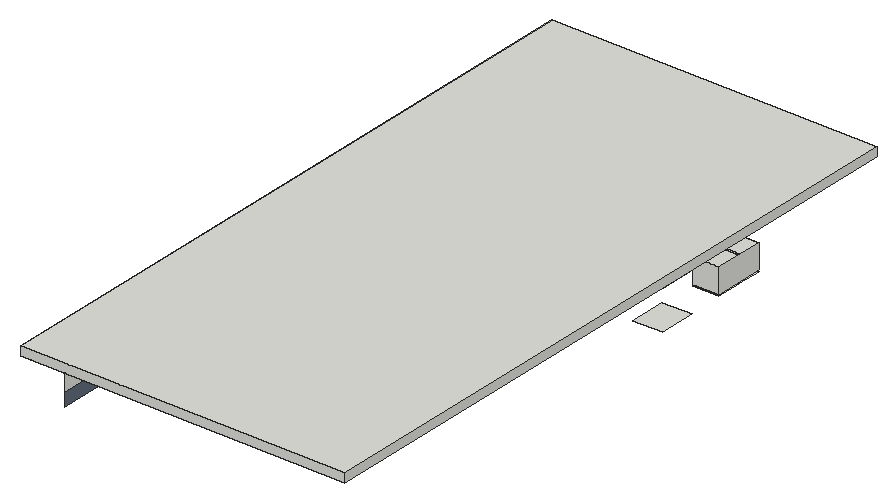
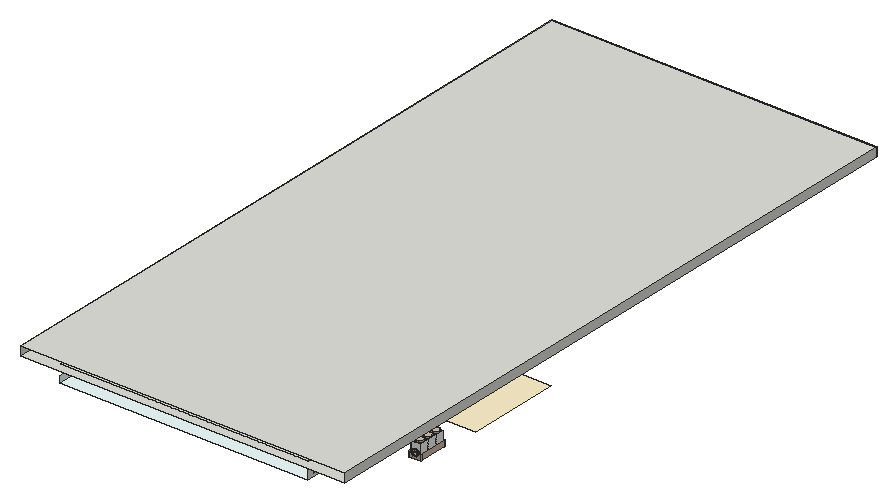
# SketchUp Ruby script. Lengths in inches.
U = 1.inch
M = Sketchup.active_model
def pt(a) = Geom::Point3d.new(a.map { |v| v * U })
def face(e, loops, mat)
  f = e.add_face(loops[0].map { |a| pt(a) })
  loops[1..].each { |l| e.add_face(l.map { |a| pt(a) }).erase! }
  f.material = f.back_material = mat if mat
  f
end
# faces: each face lists its corners as indices into pts; further lists are holes
def faces(e, pts, list, mat = nil) = list.each { |f| face(e, (f[0].is_a?(Array) ? f : [f]).map { |l| l.map { |i| pts[i] } }, mat) }
# xy, xz, yz: faces in a plane at the given z, y or x. An outline is a flat list of corners, or four numbers for a rectangle; further outlines are holes
def ring(l) = l.size == 4 ? [[l[0], l[1]], [l[2], l[1]], [l[2], l[3]], [l[0], l[3]]] : l.each_slice(2).to_a
def flat(e, list, mat, &to3) = list.each { |f| face(e, (f[0].is_a?(Array) ? f : [f]).map { |l| ring(l).map { |u, v| to3.(u, v) } }, mat) }
def xy(e, z, list, mat = nil) = flat(e, list, mat) { |x, y| [x, y, z] }
def xz(e, y, list, mat = nil) = flat(e, list, mat) { |x, z| [x, y, z] }
def yz(e, x, list, mat = nil) = flat(e, list, mat) { |y, z| [x, y, z] }
def lines(e, pts, list) = list.each { |a, b| e.add_line(pt(pts[a]), pt(pts[b])) }
# prism: a flat outline (further loops are holes) pulled along v
def prism(e, loops, v, mat = nil)
  f = face(e, loops, mat); d = Geom::Vector3d.new(v.map { |x| x * U })
  f.pushpull(f.normal.samedirection?(d) ? d.length : -d.length)
end
def box(e, o, s, mat = nil) = prism(e, [[o, [o[0] + s[0], o[1], o[2]], [o[0] + s[0], o[1] + s[1], o[2]], [o[0], o[1] + s[1], o[2]]]], [0, 0, s[2]], mat)
def at(x, y, z, deg = 0) = Geom::Transformation.translation(pt([x, y, z])) * Geom::Transformation.rotation(ORIGIN, Z_AXIS, deg.degrees)
def axes(o, x, y, z) = Geom::Transformation.new([*x, 0, *y, 0, *z, 0, *pt(o).to_a, 1])
def part(name) = M.definitions.add(name)
# library, detail: a bought-in or finely detailed component or shape, given as its bounding box
def library(name, o, s) = part(name).tap { |d| box(d.entities, o, s) }
def detail(e, o, s) = box(e.add_group.entities, o, s)
def put(e, d, t, mat = nil) = e.add_instance(d, t).tap { |i| i.material = mat if mat }
def group(e, t, mat = nil) = e.add_group.tap { |g| g.transformation = t; g.material = mat if mat }.entities
root = M.entities
M.materials.add("Branco").color = [247, 247, 247]
M.materials.add("Etiqueta").color = [244, 244, 244]
M.materials.add("Madeira").color = [213, 194, 177]
M.materials.add("[0092_Azure]").color = [240, 255, 255]
M.materials.add("[0099_LightSteelBlue]").color = [99, 110, 124]
M.materials.add("[Color D01]").color = [255, 242, 204]
M.materials.add("[Color M08]").color = [30, 30, 30]
c1 = library("10 (1)",[26.65,-5.45,122.92],[1.37,1.38,0.36])
c2 = library("Group\#125",[-0.5,-0.5,0],[1.6875,13.62,0.5625])
c3 = library("Group\#128",[-0.5,-0.5,0],[1.6875,13.62,0.5625])
c4 = library("Stocked cup rack",[0,0,0],[12.28,12.62,7.74])
c5 = library("Group\#126",[-0.5,-0.5,0],[1.6875,13.62,0.5625])
c6 = library("Group\#129",[-0.5,-0.5,0],[1.6875,13.62,0.5625])
c7 = part("Agrupar\#12")
xy(c7.entities,0,[[-280.31,0,-272.11,0.79],[0,0,0,0.79,-280.31,0.79,-280.31,161.02,0,161.02,0,161.8125,10.17,161.8125,10.17,0],[-280.31,161.02,-272.11,161.8125]],"Madeira")
xy(c7.entities,11.05,[[-272.11,11.05,0,150.76]],"Madeira")
xy(c7.entities,41.2,[[-272.11,0.79,0,11.05]],"Madeira")
xy(c7.entities,69.3,[[-272.11,150.76,0,161.02]],"Madeira")
xy(c7.entities,76.35,[[-280.31,0,-272.11,26.97],[0,0,10.17,26.97],[-280.31,134.84,-272.11,161.8125],[0,134.84,10.17,161.8125]],"Madeira")
xz(c7.entities,0,[[-280.31,0,-272.11,76.35],[0,0,10.17,76.35]],"Madeira")
xz(c7.entities,0.79,[[-272.11,0,0,41.2]],"Madeira")
xz(c7.entities,11.05,[[-272.11,11.05,0,41.2]],"Madeira")
xz(c7.entities,150.76,[[-272.11,11.05,0,69.3]],"Madeira")
xz(c7.entities,161.02,[[-272.11,0,0,69.3]],"Madeira")
xz(c7.entities,161.8125,[[-280.31,0,-272.11,76.35],[0,0,10.17,76.35]],"Madeira")
yz(c7.entities,-280.31,[[[0,0,0,76.35,26.97,76.35,31.83,88.93,32.51,90.6875,39.09,100.58,47.67,108.82,57.83,115,69.09,118.82,80.91,120.12,92.72,118.82,103.98,115,114.14,108.82,122.72,100.58,129.3,90.6875,129.98,88.93,134.84,76.35,161.8125,76.35,161.8125,0],[80.91,27.05,93.61,28.72,105.44,33.625,115.61,41.42,123.41,51.59,125.76,57.26,125.79,57.33,127.05,60.38,126.3,62.19,123.53,68.87,123.41,69.17,115.61,79.33,105.44,87.13,93.61,92.04,80.91,93.71,68.2,92.04,56.37,87.13,46.2,79.33,38.4,69.17,38.28,68.87,35.51,62.19,34.76,60.38,36.02,57.33,36.05,57.26,38.4,51.59,46.2,41.42,56.37,33.625,68.2,28.72]]],"Madeira")
yz(c7.entities,-272.11,[[[0,0,0.79,0,0.79,41.2,11.05,41.2,11.05,11.05,150.76,11.05,150.76,69.3,161.02,69.3,161.02,0,161.8125,0,161.8125,76.35,134.84,76.35,129.98,88.93,129.3,90.6875,122.72,100.58,114.14,108.82,103.98,115,92.72,118.82,80.91,120.12,69.09,118.82,57.83,115,47.67,108.82,39.09,100.58,32.51,90.6875,31.83,88.93,26.97,76.35,0,76.35],[80.91,27.05,68.2,28.72,56.37,33.625,46.2,41.42,38.4,51.59,36.05,57.26,36.02,57.33,34.76,60.38,35.51,62.19,38.28,68.87,38.4,69.17,46.2,79.33,56.37,87.13,68.2,92.04,80.91,93.71,93.61,92.04,105.44,87.13,115.61,79.33,123.41,69.17,123.53,68.87,126.3,62.19,127.05,60.38,125.79,57.33,125.76,57.26,123.41,51.59,115.61,41.42,105.44,33.625,93.61,28.72]]],"Madeira")
yz(c7.entities,0,[[[0,0,0,76.35,26.97,76.35,31.83,88.93,32.51,90.6875,39.09,100.58,47.67,108.82,57.83,115,69.09,118.82,80.91,120.12,92.72,118.82,103.98,115,114.14,108.82,122.72,100.58,129.3,90.6875,129.98,88.93,134.84,76.35,150.76,76.35,150.76,11.05,11.05,11.05,11.05,41.2,0.79,41.2,0.79,0],[80.91,27.05,93.61,28.72,105.44,33.625,115.61,41.42,123.41,51.59,125.76,57.26,125.79,57.33,127.05,60.38,126.3,62.19,123.53,68.87,123.41,69.17,115.61,79.33,105.44,87.13,93.61,92.04,80.91,93.71,68.2,92.04,56.37,87.13,46.2,79.33,38.4,69.17,38.28,68.87,35.51,62.19,34.76,60.38,36.02,57.33,36.05,57.26,38.4,51.59,46.2,41.42,56.37,33.625,68.2,28.72]],[161.02,0,161.8125,76.35],[150.76,69.3,161.02,76.35]],"Madeira")
yz(c7.entities,10.17,[[[0,0,161.8125,0,161.8125,76.35,134.84,76.35,129.98,88.93,129.3,90.6875,122.72,100.58,114.14,108.82,103.98,115,92.72,118.82,80.91,120.12,69.09,118.82,57.83,115,47.67,108.82,39.09,100.58,32.51,90.6875,31.83,88.93,26.97,76.35,0,76.35],[80.91,27.05,68.2,28.72,56.37,33.625,46.2,41.42,38.4,51.59,36.05,57.26,36.02,57.33,34.76,60.38,35.51,62.19,38.28,68.87,38.4,69.17,46.2,79.33,56.37,87.13,68.2,92.04,80.91,93.71,93.61,92.04,105.44,87.13,115.61,79.33,123.41,69.17,123.53,68.87,126.3,62.19,127.05,60.38,125.79,57.33,125.76,57.26,123.41,51.59,115.61,41.42,105.44,33.625,93.61,28.72]]],"Madeira")
p = [[-280.31,80.91,27.05],[-280.31,68.2,28.72],[-272.11,68.2,28.72],[-272.11,80.91,27.05],[10.17,68.2,28.72],[10.17,80.91,27.05],
  [0,80.91,27.05],[0,68.2,28.72],[-280.31,93.61,28.72],[-272.11,93.61,28.72],[10.17,93.61,28.72],[0,93.61,28.72],
  [-280.31,56.37,33.625],[-272.11,56.37,33.625],[10.17,56.37,33.625],[0,56.37,33.625],[-280.31,105.44,33.625],[-272.11,105.44,33.625],
  [10.17,105.44,33.625],[0,105.44,33.625],[-280.31,46.2,41.42],[-272.11,46.2,41.42],[10.17,46.2,41.42],[0,46.2,41.42],
  [-280.31,115.61,41.42],[-272.11,115.61,41.42],[10.17,115.61,41.42],[0,115.61,41.42],[-280.31,38.4,51.59],[-272.11,38.4,51.59],
  [10.17,38.4,51.59],[0,38.4,51.59],[-280.31,123.41,51.59],[-272.11,123.41,51.59],[10.17,123.41,51.59],[0,123.41,51.59],
  [-280.31,36.05,57.26],[-272.11,36.05,57.26],[10.17,36.05,57.26],[0,36.05,57.26],[-280.31,125.76,57.26],[-272.11,125.76,57.26],
  [10.17,125.76,57.26],[0,125.76,57.26],[-280.31,36.02,57.33],[-280.31,34.76,60.38],[-272.11,34.76,60.38],[-272.11,36.02,57.33],
  [10.17,34.76,60.38],[10.17,36.02,57.33],[0,36.02,57.33],[0,34.76,60.38],[-280.31,125.79,57.33],[-272.11,125.79,57.33],
  [-280.31,127.05,60.38],[-272.11,127.05,60.38],[10.17,125.79,57.33],[0,125.79,57.33],[10.17,127.05,60.38],[0,127.05,60.38],
  [-280.31,35.51,62.19],[-272.11,35.51,62.19],[10.17,35.51,62.19],[0,35.51,62.19],[-280.31,126.3,62.19],[-272.11,126.3,62.19],
  [10.17,126.3,62.19],[0,126.3,62.19],[-280.31,38.28,68.87],[-272.11,38.28,68.87],[10.17,38.28,68.87],[0,38.28,68.87],
  [-280.31,123.53,68.87],[-272.11,123.53,68.87],[10.17,123.53,68.87],[0,123.53,68.87],[-280.31,38.4,69.17],[-272.11,38.4,69.17],
  [10.17,38.4,69.17],[0,38.4,69.17],[-280.31,123.41,69.17],[-272.11,123.41,69.17],[10.17,123.41,69.17],[0,123.41,69.17],
  [-280.31,46.2,79.33],[-272.11,46.2,79.33],[10.17,46.2,79.33],[0,46.2,79.33],[-280.31,115.61,79.33],[-272.11,115.61,79.33],
  [10.17,115.61,79.33],[0,115.61,79.33],[-280.31,31.83,88.93],[-280.31,26.97,76.35],[-272.11,26.97,76.35],[-272.11,31.83,88.93],
  [10.17,26.97,76.35],[10.17,31.83,88.93],[0,31.83,88.93],[0,26.97,76.35],[-280.31,134.84,76.35],[-280.31,129.98,88.93],
  [-272.11,129.98,88.93],[-272.11,134.84,76.35],[10.17,129.98,88.93],[10.17,134.84,76.35],[0,134.84,76.35],[0,129.98,88.93],
  [-280.31,56.37,87.13],[-272.11,56.37,87.13],[10.17,56.37,87.13],[0,56.37,87.13],[-280.31,105.44,87.13],[-272.11,105.44,87.13],
  [10.17,105.44,87.13],[0,105.44,87.13],[-280.31,68.2,92.04],[-272.11,68.2,92.04],[10.17,68.2,92.04],[0,68.2,92.04],
  [-280.31,93.61,92.04],[-272.11,93.61,92.04],[10.17,93.61,92.04],[0,93.61,92.04],[-280.31,32.51,90.6875],[-272.11,32.51,90.6875],
  [10.17,32.51,90.6875],[0,32.51,90.6875],[-280.31,129.3,90.6875],[-272.11,129.3,90.6875],[10.17,129.3,90.6875],[0,129.3,90.6875],
  [-280.31,39.09,100.58],[-272.11,39.09,100.58],[10.17,39.09,100.58],[0,39.09,100.58],[-280.31,122.72,100.58],[-272.11,122.72,100.58],
  [10.17,122.72,100.58],[0,122.72,100.58],[-280.31,80.91,93.71],[-272.11,80.91,93.71],[10.17,80.91,93.71],[0,80.91,93.71],
  [-280.31,47.67,108.82],[-272.11,47.67,108.82],[10.17,47.67,108.82],[0,47.67,108.82],[-280.31,114.14,108.82],[-272.11,114.14,108.82],
  [10.17,114.14,108.82],[0,114.14,108.82],[-280.31,57.83,115],[-272.11,57.83,115],[10.17,57.83,115],[0,57.83,115],
  [-280.31,103.98,115],[-272.11,103.98,115],[10.17,103.98,115],[0,103.98,115],[-280.31,69.09,118.82],[-272.11,69.09,118.82],
  [10.17,69.09,118.82],[0,69.09,118.82],[-280.31,92.72,118.82],[-272.11,92.72,118.82],[10.17,92.72,118.82],[0,92.72,118.82],
  [-280.31,80.91,120.12],[-272.11,80.91,120.12],[10.17,80.91,120.12],[0,80.91,120.12],[-272.11,150.76,11.05],[-272.11,150.76,0],
  [-272.11,11.05,11.05],[-272.11,11.05,0]]
faces(c7.entities,p,[[0,1,2,3],[4,5,6,7],[8,0,3,9],[5,10,11,6],[1,12,13,2],[14,4,7,15],[16,8,9,17],[10,18,19,11],
  [12,20,21,13],[22,14,15,23],[24,16,17,25],[18,26,27,19],[20,28,29,21],[30,22,23,31],[32,24,25,33],[26,34,35,27],
  [28,36,37,29],[38,30,31,39],[40,32,33,41],[34,42,43,35],[44,45,46,47],[48,49,50,51],[36,44,47,37],[49,38,39,50],
  [52,40,41,53],[54,52,53,55],[42,56,57,43],[56,58,59,57],[45,60,61,46],[62,48,51,63],[64,54,55,65],[58,66,67,59],
  [60,68,69,61],[70,62,63,71],[72,64,65,73],[66,74,75,67],[68,76,77,69],[78,70,71,79],[80,72,73,81],[74,82,83,75],
  [76,84,85,77],[86,78,79,87],[88,80,81,89],[82,90,91,83],[92,93,94,95],[96,97,98,99],[100,101,102,103],[104,105,106,107],
  [84,108,109,85],[110,86,87,111],[112,88,89,113],[90,114,115,91],[108,116,117,109],[118,110,111,119],[120,112,113,121],[114,122,123,115],
  [124,92,95,125],[97,126,127,98],[101,128,129,102],[130,104,107,131],[132,124,125,133],[126,134,135,127],[128,136,137,129],[138,130,131,139],
  [116,140,141,117],[142,118,119,143],[140,120,121,141],[122,142,143,123],[144,132,133,145],[134,146,147,135],[136,148,149,137],[150,138,139,151],
  [152,144,145,153],[146,154,155,147],[148,156,157,149],[158,150,151,159],[160,152,153,161],[154,162,163,155],[156,164,165,157],[166,158,159,167],
  [168,160,161,169],[162,170,171,163],[164,168,169,165],[170,166,167,171]],"Madeira")
lines(c7.entities,p,[[172,173],[174,175]])
c8 = part("Agrupar\#11")
xy(c8.entities,0,[[0,0,86.61,89.37]],"Branco")
xy(c8.entities,123.62,[[[0,0,86.61,89.37],[43.18,1.77,6.08,23.34,6.14,44.69,6.21,66.25,43.31,87.52,43.43,87.6,80.53,66.03,80.47,44.69,80.41,23.12,43.31,1.85]]],"Branco")
xy(c8.entities,138.1875,[[43.18,1.77,43.31,1.85,80.41,23.12,80.47,44.69,80.53,66.03,43.43,87.6,43.31,87.52,6.21,66.25,6.14,44.69,6.08,23.34]],"Madeira")
xz(c8.entities,0,[[0,0,86.61,123.62]],"Etiqueta")
xz(c8.entities,89.37,[[0,0,86.61,123.62]],"Branco")
yz(c8.entities,0,[[0,0,89.37,123.62]],"Branco")
yz(c8.entities,86.61,[[0,0,89.37,123.62]],"Branco")
p = [[6.08,23.34,123.62],[43.18,1.77,123.62],[43.18,1.77,138.1875],[6.08,23.34,138.1875],[43.31,1.85,123.62],[80.41,23.12,123.62],
  [80.41,23.12,138.1875],[43.31,1.85,138.1875],[80.47,44.69,123.62],[80.53,66.03,123.62],[80.53,66.03,138.1875],[80.47,44.69,138.1875],
  [6.21,66.25,123.62],[6.14,44.69,123.62],[6.14,44.69,138.1875],[6.21,66.25,138.1875],[43.43,87.6,123.62],[43.43,87.6,138.1875],
  [43.31,87.52,123.62],[43.31,87.52,138.1875]]
faces(c8.entities,p,[[0,1,2,3],[1,4,5,6,7,2],[5,8,9,10,11,6],[12,13,0,3,14,15],[9,16,17,10],[16,18,12,15,19,17]],"Madeira")
c9 = part("Agrupar\#10")
xy(c9.entities,0,[[0,0,86.61,89.37]],"Branco")
xy(c9.entities,123.62,[[[0,0,86.61,89.37],[43.18,1.77,6.08,23.34,6.14,44.69,6.21,66.25,43.31,87.52,43.43,87.6,80.53,66.03,80.47,44.69,80.41,23.12,43.31,1.85]]],"Branco")
xy(c9.entities,138.1875,[[43.18,1.77,43.31,1.85,80.41,23.12,80.47,44.69,80.53,66.03,43.43,87.6,43.31,87.52,6.21,66.25,6.14,44.69,6.08,23.34]],"Madeira")
xz(c9.entities,0,[[0,0,86.61,123.62]],"Etiqueta")
xz(c9.entities,89.37,[[0,0,86.61,123.62]],"Branco")
yz(c9.entities,0,[[0,0,89.37,123.62]],"Branco")
yz(c9.entities,86.61,[[0,0,89.37,123.62]],"Branco")
p = [[6.08,23.34,123.62],[43.18,1.77,123.62],[43.18,1.77,138.1875],[6.08,23.34,138.1875],[43.31,1.85,123.62],[80.41,23.12,123.62],
  [80.41,23.12,138.1875],[43.31,1.85,138.1875],[80.47,44.69,123.62],[80.53,66.03,123.62],[80.53,66.03,138.1875],[80.47,44.69,138.1875],
  [6.21,66.25,123.62],[6.14,44.69,123.62],[6.14,44.69,138.1875],[6.21,66.25,138.1875],[43.43,87.6,123.62],[43.43,87.6,138.1875],
  [43.31,87.52,123.62],[43.31,87.52,138.1875]]
faces(c9.entities,p,[[0,1,2,3],[1,4,5,6,7,2],[5,8,9,10,11,6],[12,13,0,3,14,15],[9,16,17,10],[16,18,12,15,19,17]],"Madeira")
c10 = part("Agrupar\#9")
xy(c10.entities,0,[[0,0,86.61,89.37]],"Branco")
xy(c10.entities,123.62,[[[0,0,86.61,89.37],[43.18,1.77,6.08,23.34,6.14,44.69,6.21,66.25,43.31,87.52,43.43,87.6,80.53,66.03,80.47,44.69,80.41,23.12,43.31,1.85]]],"Branco")
xy(c10.entities,138.1875,[[43.18,1.77,43.31,1.85,80.41,23.12,80.47,44.69,80.53,66.03,43.43,87.6,43.31,87.52,6.21,66.25,6.14,44.69,6.08,23.34]],"Madeira")
xz(c10.entities,0,[[0,0,86.61,123.62]],"Etiqueta")
xz(c10.entities,89.37,[[0,0,86.61,123.62]],"Branco")
yz(c10.entities,0,[[0,0,89.37,123.62]],"Branco")
yz(c10.entities,86.61,[[0,0,89.37,123.62]],"Branco")
p = [[6.08,23.34,123.62],[43.18,1.77,123.62],[43.18,1.77,138.1875],[6.08,23.34,138.1875],[43.31,1.85,123.62],[80.41,23.12,123.62],
  [80.41,23.12,138.1875],[43.31,1.85,138.1875],[80.47,44.69,123.62],[80.53,66.03,123.62],[80.53,66.03,138.1875],[80.47,44.69,138.1875],
  [6.21,66.25,123.62],[6.14,44.69,123.62],[6.14,44.69,138.1875],[6.21,66.25,138.1875],[43.43,87.6,123.62],[43.43,87.6,138.1875],
  [43.31,87.52,123.62],[43.31,87.52,138.1875]]
faces(c10.entities,p,[[0,1,2,3],[1,4,5,6,7,2],[5,8,9,10,11,6],[12,13,0,3,14,15],[9,16,17,10],[16,18,12,15,19,17]],"Madeira")
c11 = part("TDS")
put(c11.entities,c7,axes([280.31,0,0],[1,0,0],[0,0.66912,0],[0,0,0.67]))
put(c11.entities,c8,at(191.09,9.47,11.02))
put(c11.entities,c9,at(100.9375,9.47,11.02))
put(c11.entities,c10,at(9.6,9.47,11.02))
c12 = part("jar")
put(c12.entities,c11,at(-649.15,-679.88,0))
xy(root,90.38,[[198,322.54,215.4375,339.38],[198,339.38,215.4375,339.91],[198,339.91,215.4375,356]])
xy(root,91.04,[[198,322.54,215.4375,356]])
xy(root,91.77,[[198,271.14,218.5625,296.01]])
xy(root,98.53,[[4.125,270.68,30,334.44]],"[Color D01]")
xy(root,100.15,[[198,297.04,198.3125,321.9]])
xy(root,100.71,[[198,297.04,198.3125,321.9]])
xy(root,107.95,[[198,322.54,215.4375,339.38],[198,339.38,215.4375,339.91],[198,339.91,215.4375,356]])
xy(root,108.59,[[198,356.64,198.3,356.94]])
xy(root,108.59,[[[30,270.125,198,444.125],[50,290.125,178,424.125]],[[50,290.125,178,424.125],[64.57,304.7,163.43,409.55],[56.1,354.125,56.87,354.25,57.58,354.58,58.19,355.07,58.65,355.71,58.92,356.44,59,357.22,58.87,358,58.55,358.71,58.05,359.31,57.41,359.77,56.68,360.05,55.9,360.125,55.13,360,54.42,359.67,53.81,359.18,53.35,358.54,53.08,357.81,53,357.03,53.13,356.25,53.45,355.54,53.95,354.94,54.59,354.48,55.32,354.2],[114,293.125,114.78,293.23,115.5,293.53,116.12,294,116.6,294.625,116.9,295.35,117,296.125,116.9,296.9,116.6,297.625,116.12,298.25,115.5,298.72,114.78,299.02,114,299.125,113.22,299.02,112.5,298.72,111.88,298.25,111.4,297.625,111.1,296.9,111,296.125,111.1,295.35,111.4,294.625,111.88,294,112.5,293.53,113.22,293.23],[114,415.125,114.78,415.23,115.5,415.53,116.12,416,116.6,416.625,116.9,417.35,117,418.125,116.9,418.9,116.6,419.625,116.12,420.25,115.5,420.72,114.78,421.02,114,421.125,113.22,421.02,112.5,420.72,111.88,420.25,111.4,419.625,111.1,418.9,111,418.125,111.1,417.35,111.4,416.625,111.88,416,112.5,415.53,113.22,415.23],[172,354.125,172.78,354.23,173.5,354.53,174.12,355,174.6,355.625,174.9,356.35,175,357.125,174.9,357.9,174.6,358.625,174.12,359.25,173.5,359.72,172.78,360.02,172,360.125,171.22,360.02,170.5,359.72,169.88,359.25,169.4,358.625,169.1,357.9,169,357.125,169.1,356.35,169.4,355.625,169.88,355,170.5,354.53,171.22,354.23],[172,415.125,172.78,415.23,173.5,415.53,174.12,416,174.6,416.625,174.9,417.35,175,418.125,174.9,418.9,174.6,419.625,174.12,420.25,173.5,420.72,172.78,421.02,172,421.125,171.22,421.02,170.5,420.72,169.88,420.25,169.4,419.625,169.1,418.9,169,418.125,169.1,417.35,169.4,416.625,169.88,416,170.5,415.53,171.22,415.23],[56,293.125,56.78,293.23,57.5,293.53,58.12,294,58.6,294.625,58.9,295.35,59,296.125,58.9,296.9,58.6,297.625,58.12,298.25,57.5,298.72,56.78,299.02,56,299.125,55.22,299.02,54.5,298.72,53.88,298.25,53.4,297.625,53.1,296.9,53,296.125,53.1,295.35,53.4,294.625,53.88,294,54.5,293.53,55.22,293.23],[171.9,293.125,172.67,293.2,173.41,293.48,174.05,293.93,174.54,294.54,174.87,295.25,175,296.02,174.92,296.8,174.65,297.53,174.19,298.17,173.59,298.67,172.88,298.99,172.1,299.125,171.33,299.05,170.59,298.77,169.95,298.32,169.46,297.71,169.13,297,169,296.23,169.08,295.45,169.35,294.72,169.81,294.08,170.41,293.58,171.12,293.26],[56.24,415.45,56.92,415.6,57.54,415.92,58.06,416.4,58.4375,416.99,58.65,417.66,58.68,418.36,58.53,419.05,58.2,419.67,57.73,420.18,57.13,420.5625,56.47,420.77,55.76,420.8,55.08,420.65,54.46,420.33,53.94,419.85,53.5625,419.26,53.35,418.59,53.32,417.89,53.47,417.2,53.8,416.58,54.27,416.07,54.87,415.6875,55.53,415.48]],[[67.14,307.26,160.86,406.99],[77.14,319.26,77.83,319.26,77.83,390.24,77.08,390.24,77.08,382.37,77.14,382.37],[150.17,319.26,150.86,390.87]],[77.14,319.26,77.83,331.88],[150.17,319.26,150.86,331.88],
  [77.14,344.5,77.83,357.125],[150.17,344.5,150.86,357.125]],"[0092_Azure]")
xy(root,108.59,[[77.14,331.88,77.83,344.5],[150.17,331.88,150.86,344.5]],"[Color M08]")
xy(root,109.47,[[67.14,307.26,160.86,308.76]],"[0092_Azure]")
xy(root,109.59,[[56,293.125,55.22,293.23,54.5,293.53,53.88,294,53.4,294.625,53.1,295.35,53,296.125,53.1,296.9,53.4,297.625,53.88,298.25,54.5,298.72,55.22,299.02,56,299.125,56.78,299.02,57.5,298.72,58.12,298.25,58.6,297.625,58.9,296.9,59,296.125,58.9,295.35,58.6,294.625,58.12,294,57.5,293.53,56.78,293.23],[114,293.125,113.22,293.23,112.5,293.53,111.88,294,111.4,294.625,111.1,295.35,111,296.125,111.1,296.9,111.4,297.625,111.88,298.25,112.5,298.72,113.22,299.02,114,299.125,114.78,299.02,115.5,298.72,116.12,298.25,116.6,297.625,116.9,296.9,117,296.125,116.9,295.35,116.6,294.625,116.12,294,115.5,293.53,114.78,293.23],[171.9,293.125,171.12,293.26,170.41,293.58,169.81,294.08,169.35,294.72,169.08,295.45,169,296.23,169.13,297,169.46,297.71,169.95,298.32,170.59,298.77,171.33,299.05,172.1,299.125,172.88,298.99,173.59,298.67,174.19,298.17,174.65,297.53,174.92,296.8,175,296.02,174.87,295.25,174.54,294.54,174.05,293.93,173.41,293.48,172.67,293.2]],"[0092_Azure]")
xy(root,120,[[0,0,0,450.125,220,450.125,220,0,198,0,198,444.125,30,444.125,30,0],[30,0,198,444.125]])
xy(root,126,[[0,0,220,450.125]])
xz(root,0,[[0,120,220,126]])
xz(root,270.125,[[30,108.59,198,112.59]],"[0092_Azure]")
xz(root,297.04,[[198,100.15,198.3125,100.71]])
xz(root,304.7,[[64.57,108.59,163.43,110.59]],"[0092_Azure]")
xz(root,307.26,[[67.14,108.59,160.86,109.47]],"[0092_Azure]")
xz(root,319.26,[[150.17,108.03,150.86,108.59]],"[0092_Azure]")
xz(root,321.9,[[198,100.15,198.3125,100.71]])
xz(root,322.54,[[198,91.04,215.4375,107.95]])
xz(root,331.88,[[77.14,108.03,77.83,108.59],[150.17,108.03,150.86,108.59]],"[0092_Azure]")
xz(root,344.5,[[150.17,108.03,150.86,108.59]],"[0092_Azure]")
xz(root,356,[[198,91.04,215.4375,107.95]])
xz(root,357.125,[[77.14,108.03,77.83,108.59],[150.17,108.03,150.86,108.59]],"[0092_Azure]")
yz(root,0,[[0,120,450.125,126]])
yz(root,30,[[0,108.59,444.125,120]])
yz(root,30,[[270.125,108.59,444.125,112.59]],"[0092_Azure]")
yz(root,30,[[0,99.09,335,108.59]],"[0099_LightSteelBlue]")
yz(root,67.14,[[307.26,108.59,406.99,109.47]],"[0092_Azure]")
yz(root,160.86,[[307.26,108.59,406.99,109.47]],"[0092_Azure]")
yz(root,198,[[270.125,108.59,444.125,112.59]],"[0092_Azure]")
yz(root,198.3125,[[297.04,100.15,321.9,100.71]])
yz(root,215.4375,[[322.54,91.04,356,107.95]])
yz(root,220,[[0,120,450.125,126]])
p = [[56,293.125,108.59],[55.22,293.23,108.59],[55.22,293.23,109.59],[56,293.125,109.59],[56.78,293.23,108.59],[56.78,293.23,109.59],
  [114,293.125,108.59],[113.22,293.23,108.59],[113.22,293.23,109.59],[114,293.125,109.59],[114.78,293.23,108.59],[114.78,293.23,109.59],
  [171.9,293.125,108.59],[171.12,293.26,108.59],[171.12,293.26,109.59],[171.9,293.125,109.59],[172.67,293.2,108.59],[172.67,293.2,109.59],
  [54.5,293.53,108.59],[54.5,293.53,109.59],[57.5,293.53,108.59],[57.5,293.53,109.59],[112.5,293.53,108.59],[112.5,293.53,109.59],
  [115.5,293.53,108.59],[115.5,293.53,109.59],[173.41,293.48,108.59],[173.41,293.48,109.59],[170.41,293.58,108.59],[170.41,293.58,109.59],
  [53.88,294,108.59],[53.88,294,109.59],[58.12,294,108.59],[58.12,294,109.59],[111.88,294,108.59],[111.88,294,109.59],
  [116.12,294,108.59],[116.12,294,109.59],[174.05,293.93,108.59],[174.05,293.93,109.59],[169.81,294.08,108.59],[169.81,294.08,109.59],
  [174.54,294.54,108.59],[174.54,294.54,109.59],[53.4,294.625,108.59],[53.4,294.625,109.59],[58.6,294.625,108.59],[58.6,294.625,109.59],
  [111.4,294.625,108.59],[111.4,294.625,109.59],[116.6,294.625,108.59],[116.6,294.625,109.59],[169.35,294.72,108.59],[169.35,294.72,109.59],
  [174.87,295.25,108.59],[174.87,295.25,109.59],[53.1,295.35,108.59],[53.1,295.35,109.59],[58.9,295.35,108.59],[58.9,295.35,109.59],
  [111.1,295.35,108.59],[111.1,295.35,109.59],[116.9,295.35,108.59],[116.9,295.35,109.59],[169.08,295.45,108.59],[169.08,295.45,109.59],
  [175,296.02,108.59],[175,296.02,109.59],[53,296.125,108.59],[53,296.125,109.59],[59,296.125,108.59],[59,296.125,109.59],
  [111,296.125,108.59],[111,296.125,109.59],[117,296.125,108.59],[117,296.125,109.59],[169,296.23,108.59],[169,296.23,109.59],
  [174.92,296.8,108.59],[174.92,296.8,109.59],[53.1,296.9,108.59],[53.1,296.9,109.59],[58.9,296.9,108.59],[58.9,296.9,109.59],
  [111.1,296.9,108.59],[111.1,296.9,109.59],[116.9,296.9,108.59],[116.9,296.9,109.59],[169.13,297,108.59],[169.13,297,109.59],
  [174.65,297.53,108.59],[174.65,297.53,109.59],[53.4,297.625,108.59],[53.4,297.625,109.59],[58.6,297.625,108.59],[58.6,297.625,109.59],
  [111.4,297.625,108.59],[111.4,297.625,109.59],[116.6,297.625,108.59],[116.6,297.625,109.59],[169.46,297.71,108.59],[169.46,297.71,109.59],
  [174.19,298.17,108.59],[174.19,298.17,109.59],[53.88,298.25,108.59],[53.88,298.25,109.59],[58.12,298.25,108.59],[58.12,298.25,109.59],
  [111.88,298.25,108.59],[111.88,298.25,109.59],[116.12,298.25,108.59],[116.12,298.25,109.59],[169.95,298.32,108.59],[169.95,298.32,109.59],
  [54.5,298.72,108.59],[54.5,298.72,109.59],[57.5,298.72,108.59],[57.5,298.72,109.59],[112.5,298.72,108.59],[112.5,298.72,109.59],
  [115.5,298.72,108.59],[115.5,298.72,109.59],[173.59,298.67,108.59],[173.59,298.67,109.59],[170.59,298.77,108.59],[170.59,298.77,109.59],
  [55.22,299.02,108.59],[55.22,299.02,109.59],[56.78,299.02,108.59],[56.78,299.02,109.59],[113.22,299.02,108.59],[113.22,299.02,109.59],
  [114.78,299.02,108.59],[114.78,299.02,109.59],[172.88,298.99,108.59],[172.88,298.99,109.59],[171.33,299.05,108.59],[171.33,299.05,109.59],
  [56,299.125,108.59],[56,299.125,109.59],[114,299.125,108.59],[114,299.125,109.59],[172.1,299.125,108.59],[172.1,299.125,109.59],
  [56.1,354.125,108.59],[55.32,354.2,108.59],[55.32,354.2,109.59],[56.1,354.125,109.59],[56.87,354.25,108.59],[56.87,354.25,109.59],
  [172,354.125,108.59],[171.22,354.23,108.59],[171.22,354.23,109.59],[172,354.125,109.59],[172.78,354.23,108.59],[172.78,354.23,109.59],
  [54.59,354.48,108.59],[54.59,354.48,109.59],[170.5,354.53,108.59],[170.5,354.53,109.59],[173.5,354.53,108.59],[173.5,354.53,109.59],
  [57.58,354.58,108.59],[57.58,354.58,109.59],[53.95,354.94,108.59],[53.95,354.94,109.59],[169.88,355,108.59],[169.88,355,109.59],
  [174.12,355,108.59],[174.12,355,109.59],[58.19,355.07,108.59],[58.19,355.07,109.59],[53.45,355.54,108.59],[53.45,355.54,109.59],
  [169.4,355.625,108.59],[169.4,355.625,109.59],[174.6,355.625,108.59],[174.6,355.625,109.59],[58.65,355.71,108.59],[58.65,355.71,109.59],
  [53.13,356.25,108.59],[53.13,356.25,109.59],[169.1,356.35,108.59],[169.1,356.35,109.59],[174.9,356.35,108.59],[174.9,356.35,109.59],
  [58.92,356.44,108.59],[58.92,356.44,109.59],[53,357.03,108.59],[53,357.03,109.59],[169,357.125,108.59],[169,357.125,109.59],
  [175,357.125,108.59],[175,357.125,109.59],[59,357.22,108.59],[59,357.22,109.59]]
faces(root,p,[[0,1,2,3],[4,0,3,5],[6,7,8,9],[10,6,9,11],[12,13,14,15],[16,12,15,17],[1,18,19,2],[20,4,5,21],
  [7,22,23,8],[24,10,11,25],[26,16,17,27],[13,28,29,14],[18,30,31,19],[32,20,21,33],[22,34,35,23],[36,24,25,37],
  [38,26,27,39],[28,40,41,29],[42,38,39,43],[30,44,45,31],[46,32,33,47],[34,48,49,35],[50,36,37,51],[40,52,53,41],
  [54,42,43,55],[44,56,57,45],[58,46,47,59],[48,60,61,49],[62,50,51,63],[52,64,65,53],[66,54,55,67],[56,68,69,57],
  [70,58,59,71],[60,72,73,61],[74,62,63,75],[64,76,77,65],[78,66,67,79],[68,80,81,69],[82,70,71,83],[72,84,85,73],
  [86,74,75,87],[76,88,89,77],[90,78,79,91],[80,92,93,81],[94,82,83,95],[84,96,97,85],[98,86,87,99],[88,100,101,89],
  [102,90,91,103],[92,104,105,93],[106,94,95,107],[96,108,109,97],[110,98,99,111],[100,112,113,101],[104,114,115,105],[116,106,107,117],
  [108,118,119,109],[120,110,111,121],[122,102,103,123],[112,124,125,113],[114,126,127,115],[128,116,117,129],[118,130,131,119],[132,120,121,133],
  [134,122,123,135],[124,136,137,125],[126,138,139,127],[138,128,129,139],[130,140,141,131],[140,132,133,141],[136,142,143,137],[142,134,135,143],
  [144,145,146,147],[148,144,147,149],[150,151,152,153],[154,150,153,155],[145,156,157,146],[151,158,159,152],[160,154,155,161],[162,148,149,163],
  [156,164,165,157],[158,166,167,159],[168,160,161,169],[170,162,163,171],[164,172,173,165],[166,174,175,167],[176,168,169,177],[178,170,171,179],
  [172,180,181,173],[174,182,183,175],[184,176,177,185],[186,178,179,187],[180,188,189,181],[182,190,191,183],[192,184,185,193],[194,186,187,195]],"[0092_Azure]")
put(root,c1,axes([-11.3,315.23,-868.875],[4.58872,0,0],[0,3.9672,0],[0,0,7.9518]),"[0092_Azure]")
put(root,c1,axes([46.64,315.23,-868.875],[4.58872,0,0],[0,3.9672,0],[0,0,7.9518]),"[0092_Azure]")
put(root,c1,axes([-69.61,315.23,-868.875],[4.58872,0,0],[0,3.9672,0],[0,0,7.9518]),"[0092_Azure]")
put(root,c2,at(150.17,319.26,108.03),"[0092_Azure]")
put(root,c3,at(77.14,319.26,108.03),"[0092_Azure]")
put(root,c4,at(198,330.65,91.04))
put(root,c5,at(150.17,344.5,108.03),"[0092_Azure]")
put(root,c6,at(77.14,344.5,108.03),"[0092_Azure]")
put(root,c12,axes([-24.34,391.11,90.07],[0,0.0715,0],[-0.0715,0,0],[0,0,0.0715]))
